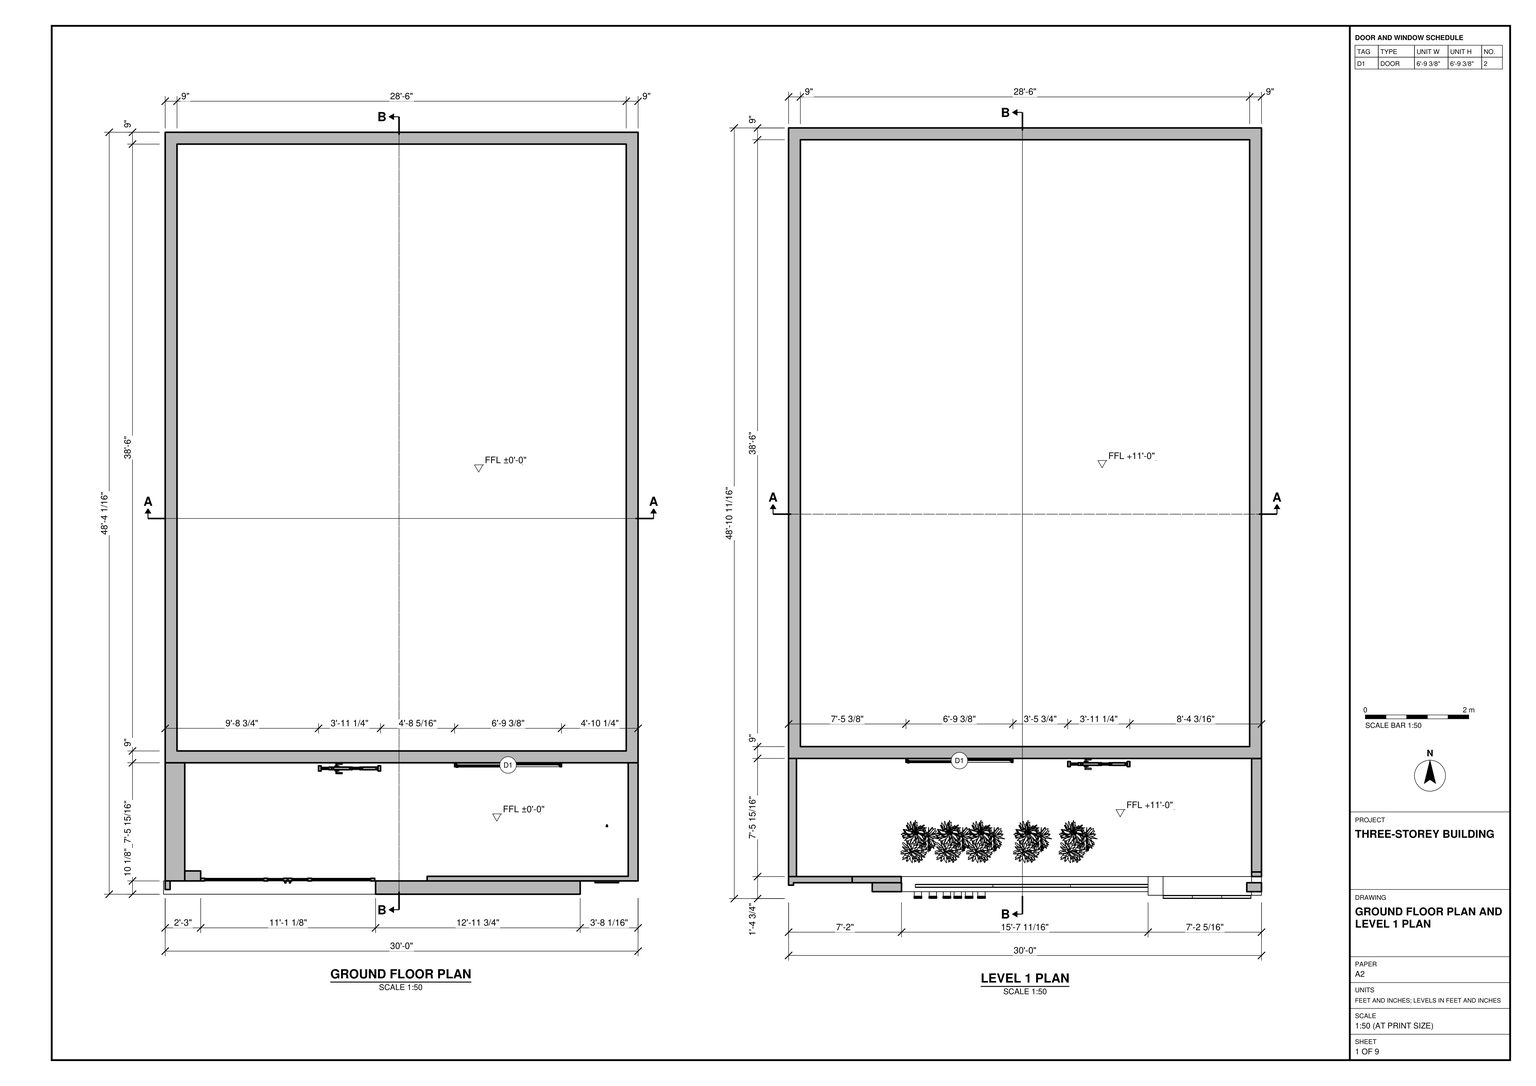
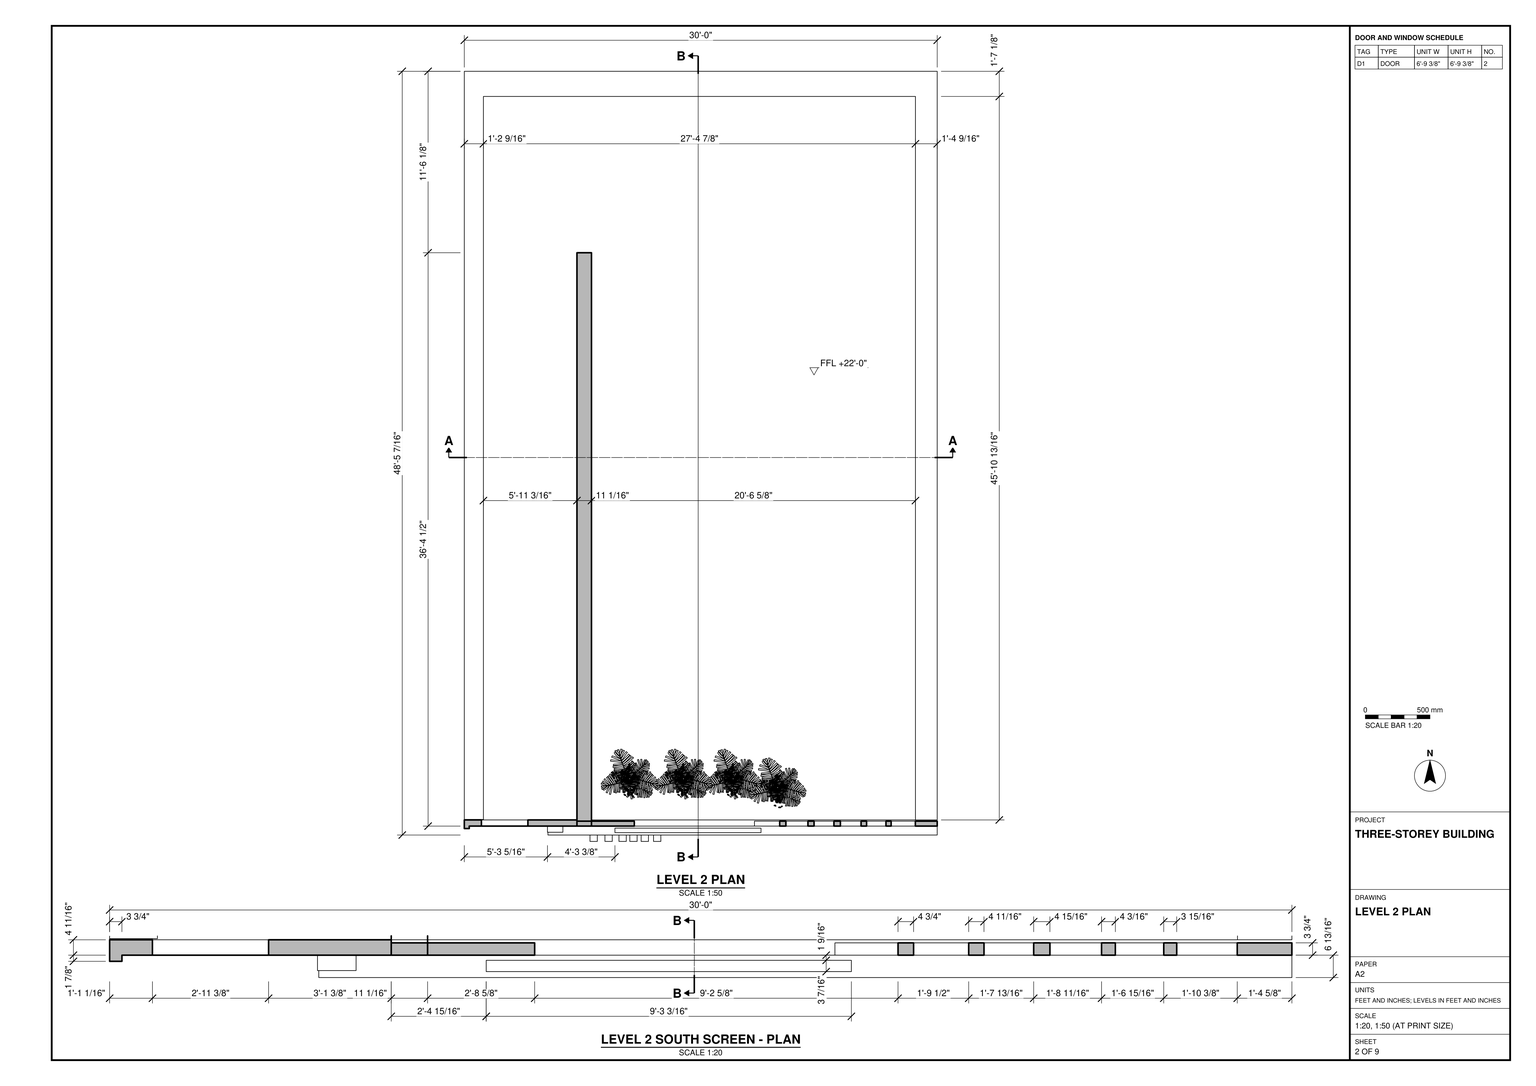
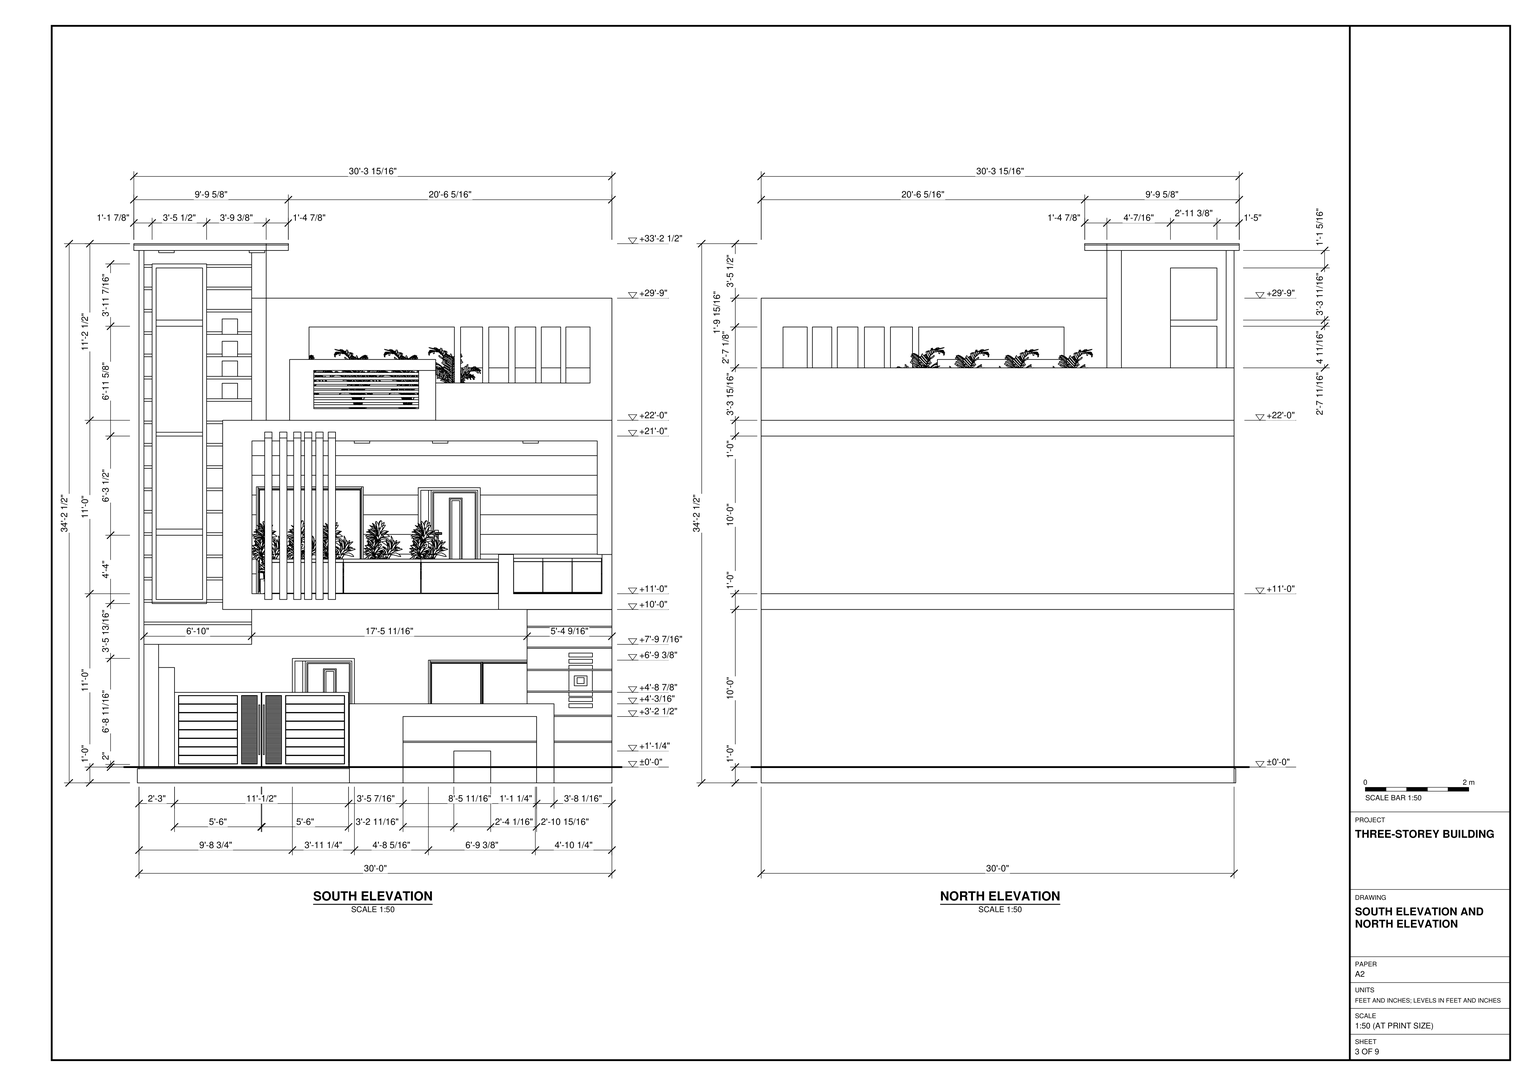
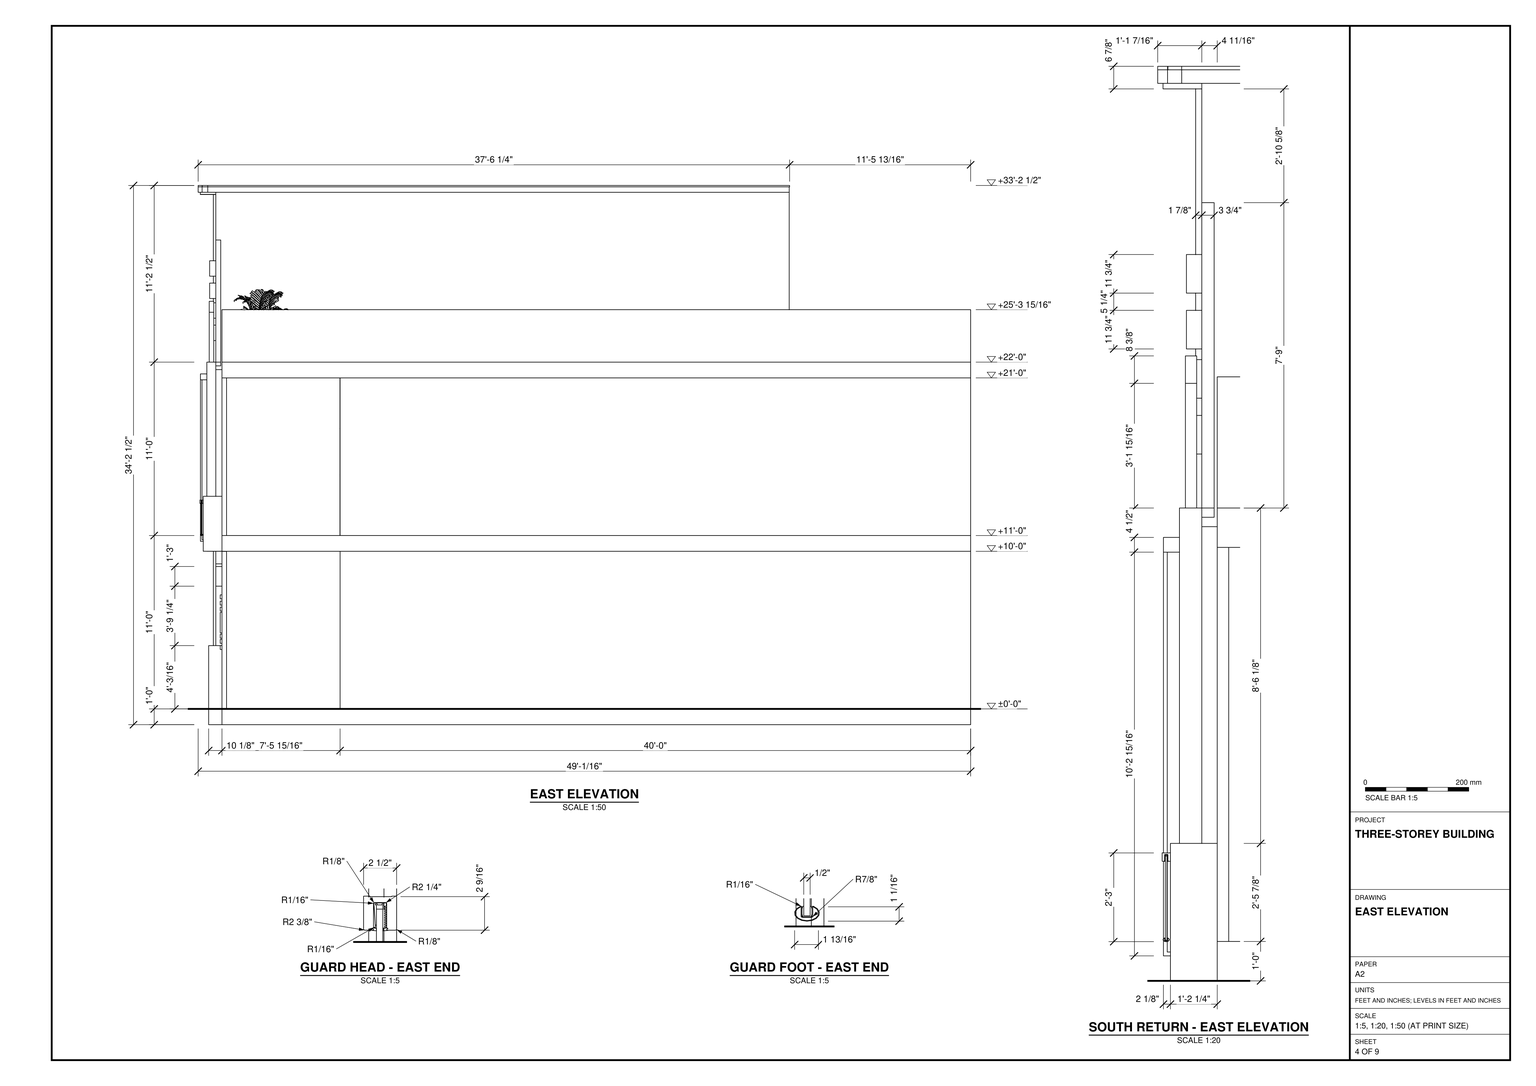
Build the three-storey building in SketchUp from task_files/diagram_01.pdf. Work in feet and inches. The overall model extents are 30'-3 15/16" wide, 49'-1/16" deep and 34'-2 1/2" high. Set the finished floor levels at ±0'-0", +11'-0" and +22'-0".

Use the plans to lay out the rectangular lower storeys with 9" perimeter walls and recessed outdoor spaces along the south side. Model the base, floor slabs and roof terrace with the edge profiles shown in elevation. At the ground-floor frontage, place the paired gate beside the low wall. Set the doors back from the gate line. The wide sliding door is on the right at ground level and on the left on the storey above when viewed from the south.

Build the projecting frame, railing and vertical fins around the first-floor balcony. On the roof terrace, include the offset longitudinal wall and the south screen with its wide opening, narrow slots and horizontal louvres. Match the tall capped bay at the west end of the south elevation. Decor and loose items, including the plants on the balcony and terrace, may be any suitable library components.

Keep shell elements such as walls, slabs and roof parts in separate groups or components, group each furniture or joinery piece separately, and use components for repeated parts. Save one SketchUp model as output_files/three_storey_building_with_a_screened_south_terrace.skp.

# SketchUp Ruby script. Lengths in inches.
U = 1.inch
M = Sketchup.active_model
def pt(a) = Geom::Point3d.new(a.map { |v| v * U })
def face(e, loops, mat)
  f = e.add_face(loops[0].map { |a| pt(a) })
  loops[1..].each { |l| e.add_face(l.map { |a| pt(a) }).erase! }
  f.material = f.back_material = mat if mat
  f
end
# faces: each face lists its corners as indices into pts; further lists are holes
def faces(e, pts, list, mat = nil) = list.each { |f| face(e, (f[0].is_a?(Array) ? f : [f]).map { |l| l.map { |i| pts[i] } }, mat) }
# xy, xz, yz: faces in a plane at the given z, y or x. An outline is a flat list of corners, or four numbers for a rectangle; further outlines are holes
def ring(l) = l.size == 4 ? [[l[0], l[1]], [l[2], l[1]], [l[2], l[3]], [l[0], l[3]]] : l.each_slice(2).to_a
def flat(e, list, mat, &to3) = list.each { |f| face(e, (f[0].is_a?(Array) ? f : [f]).map { |l| ring(l).map { |u, v| to3.(u, v) } }, mat) }
def xy(e, z, list, mat = nil) = flat(e, list, mat) { |x, y| [x, y, z] }
def xz(e, y, list, mat = nil) = flat(e, list, mat) { |x, z| [x, y, z] }
def yz(e, x, list, mat = nil) = flat(e, list, mat) { |y, z| [x, y, z] }
def lines(e, pts, list) = list.each { |a, b| e.add_line(pt(pts[a]), pt(pts[b])) }
# prism: a flat outline (further loops are holes) pulled along v
def prism(e, loops, v, mat = nil)
  f = face(e, loops, mat); d = Geom::Vector3d.new(v.map { |x| x * U })
  f.pushpull(f.normal.samedirection?(d) ? d.length : -d.length)
end
def box(e, o, s, mat = nil) = prism(e, [[o, [o[0] + s[0], o[1], o[2]], [o[0] + s[0], o[1] + s[1], o[2]], [o[0], o[1] + s[1], o[2]]]], [0, 0, s[2]], mat)
def at(x, y, z, deg = 0) = Geom::Transformation.translation(pt([x, y, z])) * Geom::Transformation.rotation(ORIGIN, Z_AXIS, deg.degrees)
def axes(o, x, y, z) = Geom::Transformation.new([*x, 0, *y, 0, *z, 0, *pt(o).to_a, 1])
def part(name) = M.definitions.add(name)
# library, detail: a bought-in or finely detailed component or shape, given as its bounding box
def library(name, o, s) = part(name).tap { |d| box(d.entities, o, s) }
def detail(e, o, s) = box(e.add_group.entities, o, s)
def put(e, d, t, mat = nil) = e.add_instance(d, t).tap { |i| i.material = mat if mat }
def group(e, t, mat = nil) = e.add_group.tap { |g| g.transformation = t; g.material = mat if mat }.entities
root = M.entities
M.materials.add("Glass_Tinted_Gray").color = [0, 0, 0]
M.materials["Glass_Tinted_Gray"].alpha = 0.125
M.materials.add("[0131_Silver]").color = [192, 192, 192]
M.materials.add("[0135_DarkGray]").color = [81, 81, 81]
M.materials.add("[Color C02]").color = [255, 204, 153]
M.materials.add("[Color C07]").color = [153, 76, 0]
M.materials.add("[Color D01]").color = [255, 242, 204]
M.materials.add("[Color E03]").color = [255, 255, 101]
M.materials.add("[Color F07]").color = [81, 104, 58]
M.materials.add("[Color M00]").color = [255, 255, 255]
M.materials.add("[Color M06]").color = [86, 86, 86]
M.materials.add("[Color M08]").color = [30, 30, 30]
M.materials.add("[Color M09]").color = [0, 0, 0]
M.materials.add("[Mirror 02]").color = [229, 229, 229]
M.materials.add("[Terrazzo Light Blue]").color = [196, 214, 227]
M.materials.add("[Translucent Glass Blue]").color = [100, 149, 237]
M.materials["[Translucent Glass Blue]"].alpha = 0.5
M.materials.add("[Wood Cherry Original]").color = [152, 86, 42]
c1 = library("ประตู",[99.61,0,0],[47.24,8.5625,80.71])
c2 = part("PENTEK_RP Fineline 50S_Sliding_DoorCase_E1")
box(c2.entities,[0,0,0],[1.51,3.66,99.27],"[0135_DarkGray]")
c3 = part("PENTEK_RP Fineline 50S_SlidingDooe_Case_E2")
box(c3.entities,[0,0,0],[96.25,3.66,1.51],"[0135_DarkGray]")
c4 = part("pentek_RP Fineline 50S_SlidingDoor_Case")
put(c4.entities,c2,at(97.76,0,0))
put(c4.entities,c3,at(1.51,0,0))
put(c4.entities,c2,at(0,0,0))
put(c4.entities,c3,at(1.51,0,97.76))
c5 = part("PENTEK_RP Fineline 50S_SlidingDoor_GlazingBead_2")
box(c5.entities,[0,0,0],[0.56,0.59,94.39],"[0135_DarkGray]")
c6 = part("PENTEK_RP Fineline 50S_SlidingDoor_Glass")
box(c6.entities,[0,0,0],[46.58,0.16,94.39],"Glass_Tinted_Gray")
c7 = part("PENTEK_RP Fineline 50S_SlidingDoor_GlazingBead")
box(c7.entities,[0,0,0],[45.47,0.59,0.56],"[0135_DarkGray]")
c8 = part("PENTEK_RP Fineline 50S_SlidingDoor_Leaf_E1")
xy(c8.entities,0,[[0,0,0.93,1.97],[0.93,1.57,1.49,1.97]],"[0135_DarkGray]")
xy(c8.entities,96.25,[[0,0,0.93,0,0.93,1.57,1.49,1.57,1.49,1.97,0,1.97]],"[0135_DarkGray]")
xz(c8.entities,0,[[0,0,0.93,96.25]],"[0135_DarkGray]")
xz(c8.entities,1.57,[[0.93,0,1.49,95.32],[0.93,95.32,1.49,96.25]],"[0135_DarkGray]")
xz(c8.entities,1.97,[[0,0,1.49,96.25]],"[0135_DarkGray]")
yz(c8.entities,0,[[0,0,1.97,96.25]],"[0135_DarkGray]")
yz(c8.entities,0.93,[[0,0,1.57,0.93],[0,0.93,1.57,95.32],[0,95.32,1.57,96.25]],"[0135_DarkGray]")
yz(c8.entities,1.49,[[1.57,0,1.97,95.32],[1.57,95.32,1.97,96.25]],"[0135_DarkGray]")
c9 = part("PENTEK_RP Fineline 50S_SlidingDoor_Leaf_E2")
xy(c9.entities,0,[[0,0,0,1.57,0.56,1.57,0.56,1.97,46.02,1.97,46.02,1.57,46.58,1.57,46.58,0]],"[0135_DarkGray]")
xy(c9.entities,0.93,[[0,0,46.58,1.57]],"[0135_DarkGray]")
xy(c9.entities,1.49,[[0.56,1.57,46.02,1.97]],"[0135_DarkGray]")
xz(c9.entities,0,[[0,0,46.58,0.93]],"[0135_DarkGray]")
xz(c9.entities,1.57,[[0,0,0.56,0.93],[46.02,0,46.58,0.93],[0.56,0.93,46.02,1.49]],"[0135_DarkGray]")
xz(c9.entities,1.97,[[0.56,0,46.02,1.49]],"[0135_DarkGray]")
yz(c9.entities,0,[[0,0,1.57,0.93]],"[0135_DarkGray]")
yz(c9.entities,0.56,[[1.57,0,1.97,0.93],[1.57,0.93,1.97,1.49]],"[0135_DarkGray]")
yz(c9.entities,46.02,[[1.57,0,1.97,0.93],[1.57,0.93,1.97,1.49]],"[0135_DarkGray]")
yz(c9.entities,46.58,[[0,0,1.57,0.93]],"[0135_DarkGray]")
c10 = part("PENTEK_RP Fineline S_SlidingDoor_Leaf1")
put(c10.entities,c5,at(0.93,0,0.93))
put(c10.entities,c5,at(46.96,0,0.93))
put(c10.entities,c6,at(1.49,1.42,0.93))
put(c10.entities,c7,at(1.49,0,0.93))
put(c10.entities,c6,at(1.49,0.59,0.93),"[Terrazzo Light Blue]")
put(c10.entities,c8,at(0,0,0))
put(c10.entities,c8,axes([48.44,0,0],[-1,0,0],[0,1,0],[0,0,1]))
put(c10.entities,c9,axes([0.93,0,96.25],[1,0,0],[0,1,0],[0,0,-1]))
put(c10.entities,c9,at(0.93,0,0))
put(c10.entities,c7,at(1.49,0,94.77))
c11 = part("PENTEK_RP Fineline 50S_SlidingDoor_Leaf2")
put(c11.entities,c6,at(1.49,1.42,0.93))
put(c11.entities,c7,at(1.49,0,94.77))
put(c11.entities,c5,at(46.96,0,0.93))
put(c11.entities,c6,at(1.49,0.59,0.93),"[Mirror 02]")
put(c11.entities,c5,at(0.93,0,0.93))
put(c11.entities,c8,at(0,0,0))
put(c11.entities,c8,axes([48.44,0,0],[-1,0,0],[0,1,0],[0,0,1]))
put(c11.entities,c7,at(1.49,0,0.93))
put(c11.entities,c9,axes([0.93,0,96.25],[1,0,0],[0,1,0],[0,0,-1]))
put(c11.entities,c9,at(0.93,0,0))
c12 = part("PENTEK - Slimmest Steel Sliding Door / Window\#1")
put(c12.entities,c4,at(0,-1.88,-0.09))
put(c12.entities,c10,at(1.51,-2.27,1.42))
put(c12.entities,c11,at(49.32,-0.3,1.42))
c13 = library("Wagner Glass Railing",[9.08,102.375,1.53],[2.51,145.5,42.05])
c14 = part("Gate+Design_02_ar+kalil")
p = [[0,0,0],[1,0,0],[1,1,0]]
lines(c14.entities,p,[[0,1],[1,2],[2,0]])
c15 = part("Gate leaf frame")
xy(c15.entities,0,[[[0,0,66,72],[3,3,48,69],[51,3,63,69]]])
xy(c15.entities,0.5,[[3,3,48,69]])
xy(c15.entities,1.5,[[3,3,48,11.25],[3,11.25,48,19.5],[3,19.5,48,27.75],[3,27.75,48,36],[3,36,48,44.25],
  [3,44.25,48,52.5],[3,52.5,48,60.75],[3,60.75,48,69]])
xy(c15.entities,2,[[[0,0,66,72],[3,3,48,69],[51,3,63,69]]])
xz(c15.entities,0,[[0,0,51,2],[51,0,66,2]])
xz(c15.entities,3,[[3,0,27,0.5],[27,0,48,0.5],[51,0,63,2],[3,1.5,48,2]])
xz(c15.entities,69,[[3,0,48,0.5],[51,0,63,2],[3,1.5,48,2]])
xz(c15.entities,72,[[0,0,66,2]])
yz(c15.entities,0,[[0,0,72,2]])
yz(c15.entities,3,[[3,0,69,0.5],[3,1.5,69,2]])
yz(c15.entities,48,[[3,0,69,0.5],[3,1.5,69,2]])
yz(c15.entities,51,[[3,0,69,2]])
yz(c15.entities,63,[[3,0,69,2]])
yz(c15.entities,66,[[0,0,72,2]])
c16 = part("Gate infill slat")
box(c16.entities,[0,0,0],[12,1,1])
c17 = part("Slatted gate infill")
put(c17.entities,c16,at(3,0.5,22.5))
put(c17.entities,c16,at(3,0.5,26.5))
put(c17.entities,c16,at(3,0.5,28.5))
put(c17.entities,c16,at(3,0.5,4.5))
put(c17.entities,c16,at(3,0.5,2.5))
put(c17.entities,c16,at(3,0.5,54.5))
put(c17.entities,c16,at(3,0.5,56.5))
put(c17.entities,c16,at(3,0.5,24.5))
put(c17.entities,c16,at(3,0.5,20.5))
put(c17.entities,c16,at(3,0.5,34.5))
put(c17.entities,c16,at(3,0.5,6.5))
put(c17.entities,c16,at(3,0.5,42.5))
put(c17.entities,c16,at(3,0.5,0.5))
put(c17.entities,c16,at(3,0.5,10.5))
put(c17.entities,c16,at(3,0.5,16.5))
put(c17.entities,c16,at(3,0.5,18.5))
put(c17.entities,c16,at(3,0.5,58.5))
put(c17.entities,c16,at(3,0.5,40.5))
put(c17.entities,c16,at(3,0.5,60.5))
put(c17.entities,c16,at(3,0.5,36.5))
put(c17.entities,c16,at(3,0.5,38.5))
put(c17.entities,c16,at(3,0.5,32.5))
put(c17.entities,c16,at(3,0.5,8.5))
put(c17.entities,c16,at(3,0.5,64.5))
put(c17.entities,c16,at(3,0.5,12.5))
put(c17.entities,c16,at(3,0.5,44.5))
put(c17.entities,c16,at(3,0.5,46.5))
put(c17.entities,c16,at(3,0.5,52.5))
put(c17.entities,c16,at(3,0.5,48.5))
put(c17.entities,c16,at(3,0.5,50.5))
put(c17.entities,c16,at(3,0.5,62.5))
put(c17.entities,c16,at(3,0.5,14.5))
put(c17.entities,c16,at(3,0.5,30.5))
c18 = part("Gate cladding strip")
xy(c18.entities,0.25,[[0.25,0,44.75,0.15]])
xy(c18.entities,8,[[0.25,0,44.75,0.15]])
xz(c18.entities,0,[[0.25,0.25,44.75,8]])
xz(c18.entities,0.15,[[[0,0,45,8.25],[0.25,0.25,44.75,8]]])
yz(c18.entities,0.25,[[0,0.25,0.15,8]])
yz(c18.entities,44.75,[[0,0.25,0.15,8]])
p = [[0,0.15,0],[0.25,0,0.25],[44.75,0,0.25],[45,0.15,0],[0,0.15,8.25],[0.25,0,8],
  [44.75,0,8],[45,0.15,8.25]]
faces(c18.entities,p,[[0,1,2,3],[4,5,1,0],[3,2,6,7],[5,4,7,6]])
c19 = part("Gate infill panel")
put(c19.entities,c18,at(0,0,24.75))
put(c19.entities,c18,at(0,0,57.75))
put(c19.entities,c18,at(0,0,49.5))
put(c19.entities,c18,at(0,0,41.25))
put(c19.entities,c18,at(0,0,33))
put(c19.entities,c18,axes([0,1.3,49.5],[1,0,0],[0,-1,0],[0,0,1]))
put(c19.entities,c18,at(0,0,16.5))
put(c19.entities,c18,at(0,0,8.25))
put(c19.entities,c18,axes([0,1.3,24.75],[1,0,0],[0,-1,0],[0,0,1]))
put(c19.entities,c18,at(0,0,0))
put(c19.entities,c18,axes([0,1.3,57.75],[1,0,0],[0,-1,0],[0,0,1]))
put(c19.entities,c18,axes([0,1.3,41.25],[1,0,0],[0,-1,0],[0,0,1]))
put(c19.entities,c18,axes([0,1.3,33],[1,0,0],[0,-1,0],[0,0,1]))
put(c19.entities,c18,axes([0,1.3,16.5],[1,0,0],[0,-1,0],[0,0,1]))
put(c19.entities,c18,axes([0,1.3,8.25],[1,0,0],[0,-1,0],[0,0,1]))
put(c19.entities,c18,axes([0,1.3,0],[1,0,0],[0,-1,0],[0,0,1]))
c20 = part("Gate leaf")
put(c20.entities,c15,axes([0,2,0],[1,0,0],[0,0,1],[0,-1,0]),"[0131_Silver]")
put(c20.entities,c17,at(48,0,3),"[0131_Silver]")
put(c20.entities,c19,at(3,0.35,3))
c21 = part("Gate pull handle")
prism(c21.entities,[[[0.35,0,3.8],[0.35,0,3],[0.35,-1.5,3],[0.35,-1.5,51],[0.35,0,51],[0.35,0,50.2],[0.35,-1,50.2],[0.35,-1,3.8]]],[0.8,0,0])
c22 = part("gate1")
put(c22.entities,c20,axes([145.27,6.5625,-22.58],[-1,0,0],[0,1,0],[0,0,1]))
put(c22.entities,c21,at(321.29,49.48,9),"[0131_Silver]")
put(c22.entities,c20,at(12.77,6.5625,-22.58))
put(c22.entities,c21,at(76.52,6.5625,-13.58),"[0131_Silver]")
put(c22.entities,c21,at(80.02,6.5625,-13.58),"[0131_Silver]")
c23 = library("KentiaPalm",[-22.86,-14.31,0],[47.49,43.96,59.125])
c24 = library("plant",[-35.72,-28.42,0],[66.31,67.39,84.38])
c25 = part("グループ\#88")
detail(c25.entities,[0,0,0],[11.8125,11.8125,1.69])
c26 = part("CL OL251733")
put(c26.entities,c25,axes([4.91,11.8125,72.56],[1,0,0],[0,-1,0],[0,0,-1]))
c27 = part("Group\#4")
box(c27.entities,[0,0,0],[5.5625,4.5,4.875])
c28 = part("Group\#5")
box(c28.entities,[0,0,0],[11.75,11.75,4.6875])
c29 = part("Group\#12")
box(c29.entities,[0,0,0],[2.125,2.125,85.0625])
prism(root,[[[3.9375,588.0625,264],[363.9375,588.0625,264],[363.9375,18.125,264],[347.375,18.125,264],[347.375,568.91,264],[18.48,568.91,264],[18.48,18.47,264],[3.9375,18.47,264]]],[0,0,39.9375])
xy(root,-12,[[2.67,8,204.92,18.125],[306.61,8,319.875,18.125],[243.61,15.8125,271.67,18.125]])
xy(root,0,[[3.9375,11.5625,7.6875,18.125],[3.9375,18.125,18.84,108.0625],[18.84,18.125,30.96,25.73],[203.36,18.125,363.9375,21.625],[356.42,21.625,363.9375,108.0625],
  [[3.9375,108.0625,363.9375,588.0625],[12.9375,117.0625,354.9375,579.0625]],[12.9375,117.0625,354.9375,579.0625]])
xy(root,12.25,[[243.61,15.8125,271.67,18.125]],"[Color C07]")
xy(root,38.52,[[204.92,8,306.61,18.125]])
xy(root,48.19,[[203.36,18.125,299.36,21.625]])
xy(root,48.19,[[164.11,8,319.875,18.125]],"[Color C07]")
xy(root,57.87,[[331.23,16.8125,349.06,18.125]])
xy(root,61.91,[[335.27,16.8125,345.01,18.125]])
xy(root,63.58,[[337.45,16.8125,342.76,18.125]])
xy(root,68.14,[[337.45,16.8125,342.76,18.125]])
xy(root,69.44,[[335.27,16.8125,345.01,18.125]])
xy(root,73.48,[[331.23,16.8125,349.06,18.125]])
xy(root,75.8125,[[18.84,18.125,30.96,25.73]],"[Color C07]")
xy(root,93.4375,[[7.6875,13.4375,7.6875,18.125,78.66,18.125,78.66,108.0625,89.69,108.0625,89.69,13.4375]])
xy(root,119.9,[[299.36,18.125,363.9375,21.625]])
xy(root,120,[[67.625,6.625,278.25,18.125],[3.9375,18.125,18.84,108.0625],[78.66,18.125,89.69,108.0625],[356.42,21.625,363.9375,108.0625],[[3.9375,108.0625,363.9375,588.0625],[12.9375,117.0625,354.9375,579.0625]]])
xy(root,120.02,[[277.62,3.875,363.9375,18.125]])
xy(root,127.58,[[16.97,13.4375,52.34,18.125]])
xy(root,127.61,[[99.61,1.75,105.18,6.625],[110.99,1.75,116.55,6.625],[121.68,1.75,127.24,6.625],[129.93,1.75,135.49,6.625],[138.55,1.75,144.11,6.625],
  [147.99,1.75,153.55,6.625]],"[Color M06]")
xy(root,128.78,[[99.61,2.91,105.18,6.625],[110.99,2.91,116.55,6.625],[121.68,2.91,127.24,6.625],[129.93,2.91,135.49,6.625],[138.55,2.91,144.11,6.625],
  [147.99,2.91,153.55,6.625]])
xy(root,131.9375,[[289.03,3.875,356.42,18.125]])
xy(root,132,[[89.92,6.625,278.25,6.625,278.25,18.125,67.625,18.125,67.625,13.4375,89.92,13.4375],[3.9375,18.125,9.95,108.0625],[356.42,18.125,363.9375,21.625],[356.42,21.625,363.9375,107.9375],[[3.9375,108.0625,363.9375,588.0625],[12.9375,117.0625,354.9375,579.0625]],
  [12.9375,117.0625,354.9375,579.0625]])
xy(root,161.86,[[277.62,3.875,289.03,18.125],[356.42,3.875,363.9375,6.625],[352.76,6.625,356.42,13.4375],[356.42,6.625,363.9375,13.4375],[356.42,13.4375,363.9375,18.125]])
xy(root,176.51,[[16.97,13.4375,52.34,18.125]])
xy(root,181.19,[[16.97,13.4375,52.34,18.125]])
xy(root,248.32,[[89.92,6.625,352.76,13.4375]],"[Wood Cherry Original]")
xy(root,250.55,[[99.61,1.75,105.18,2.91]])
xy(root,252,[[16.97,13.4375,52.34,18.125],[3.9375,18.125,9.95,108.0625],[356.42,18.125,363.9375,21.625],[356.42,21.625,363.9375,107.9375],[[3.9375,108.0625,363.9375,588.0625],[12.9375,117.0625,354.9375,579.0625]]])
xy(root,254.9,[[16.97,13.4375,52.34,18.125]])
xy(root,258.3125,[[89.69,13.4375,100.75,449.9375]])
xy(root,261.17,[[89.69,13.4375,133.36,17.1875]])
xy(root,264,[[[67.625,6.625,363.9375,13.4375],[118.61,8.4375,229.79,11.875]],[224.8,13.4375,363.9375,17.1875]])
xy(root,272.85,[[136.98,8.4375,216.82,11.875]],"[Color F07]")
xy(root,292.37,[[324.92,13.4375,328.87,17.1875],[328.87,13.4375,347.3,17.1875]])
xy(root,292.43,[[224.8,13.4375,244.01,17.1875],[244.01,13.4375,248.75,17.1875],[248.75,13.4375,265.52,17.1875],[265.52,13.4375,270.1875,17.1875],[270.1875,13.4375,285.3125,17.1875],
  [285.3125,13.4375,290.26,17.1875],[290.26,13.4375,305.98,17.1875],[305.98,13.4375,310.18,17.1875],[310.18,13.4375,324.92,17.1875]])
xy(root,301.96,[[216.82,8.4375,229.79,11.875]])
xy(root,301.96,[[136.98,8.4375,216.82,11.875]],"[Color F07]")
xy(root,310.3125,[[118.61,8.4375,229.79,11.875]],"[Color F07]")
xy(root,335.06,[[133.36,13.4375,244.01,17.1875],[248.75,13.4375,265.52,17.1875],[270.1875,13.4375,285.3125,17.1875],[290.26,13.4375,305.98,17.1875],[310.18,13.4375,324.92,17.1875],
  [328.87,13.4375,347.3,17.1875]])
xy(root,335.61,[[16.97,13.4375,52.34,18.125]])
xy(root,340.3,[[16.97,13.4375,52.34,18.125]])
xy(root,356.98,[[89.69,13.4375,363.9375,17.1875]])
xy(root,380,[[16.97,13.4375,52.34,18.125]])
xy(root,393.3125,[[0,11.5625,3.9375,13.4375],[3.9375,11.5625,7.6875,13.4375],[89.69,13.4375,100.75,449.9375]])
xy(root,393.3125,[[0,0,100.75,3],[100.75,0,117.63,3],[0,3,100.75,7.3125],[100.75,3,117.63,7.3125],[0,7.3125,0,11.5625,7.6875,11.5625,7.6875,13.4375,100.75,13.4375,100.75,7.3125],
  [100.75,7.3125,117.63,13.4375],[0,13.4375,3.9375,449.9375],[100.75,13.4375,117.63,449.9375],[3.9375,18.125,9.95,449.9375],[9.95,18.125,89.69,449.9375]],"[Color C07]")
xy(root,397.4375,[[0,0,100.75,3],[100.75,0,117.63,3],[0,3,100.75,7.3125],[100.75,3,103.75,3.125],[103.75,3,117.63,3.125],
  [100.75,3.125,117.63,7.3125],[0,7.3125,100.75,449.9375],[100.75,7.3125,117.63,449.9375],[117.63,7.3125,117.69,450.25],[100.75,449.9375,117.63,450.25]])
xy(root,398.5,[[100.75,3,103.75,3.125]])
xy(root,398.5,[[0,0,100.75,3],[100.75,0,117.63,3],[0,3,100.75,7.3125],[100.75,3.125,117.63,7.3125],[0,7.3125,100.75,449.9375],
  [100.75,7.3125,117.69,450.25]],"[Color C07]")
xz(root,0,[[0,393.3125,100.75,397.4375],[100.75,393.3125,117.63,397.4375],[0,397.4375,100.75,398.5],[100.75,397.4375,117.63,398.5]],"[Color C07]")
xz(root,1.75,[[99.61,127.61,105.18,250.55],[110.99,127.61,116.55,250.55],[121.68,127.61,127.24,250.55],[129.93,127.61,135.49,250.55],[138.55,127.61,144.11,250.55],
  [147.99,127.61,153.55,250.55]],"[Color M06]")
xz(root,2.91,[[99.61,128.78,105.18,250.55],[110.99,128.78,116.55,250.55],[121.68,128.78,127.24,250.55],[129.93,128.78,135.49,250.55],[138.55,128.78,144.11,250.55],
  [147.99,128.78,153.55,250.55]])
xz(root,3,[[0,393.3125,100.75,397.4375],[100.75,393.3125,117.63,397.4375],[0,397.4375,100.75,398.5],[100.75,397.4375,103.75,398.5],[103.75,397.4375,117.63,398.5]])
xz(root,3.125,[[103.75,397.4375,117.63,398.5]])
xz(root,3.875,[[277.62,120.02,363.9375,120.02,363.9375,161.86,356.42,161.86,356.42,131.9375,289.03,131.9375,289.03,161.86,277.62,161.86]])
xz(root,6.625,[[[67.625,120,278.25,120,278.25,132,89.92,132,89.92,248.32,352.76,248.32,352.76,161.86,363.9375,161.86,363.9375,264,67.625,264],[99.61,127.61,105.18,128.78],[121.68,127.61,127.24,128.78],[129.93,127.61,135.49,128.78],[138.55,127.61,144.11,128.78],[147.99,127.61,153.55,128.78]]],"[Color C07]")
xz(root,7.3125,[[0,393.3125,100.75,397.4375],[100.75,393.3125,117.63,397.4375],[0,397.4375,100.75,398.5],[100.75,397.4375,117.63,398.5],[117.63,397.4375,117.69,398.5]])
xz(root,8,[[164.11,-12,204.92,-12,204.92,38.52,306.61,38.52,306.61,-12,319.875,-12,319.875,48.19,164.11,48.19]],"[Color C07]")
xz(root,8.4375,[[[118.61,264,229.79,310.3125],[136.98,272.85,216.82,301.96]]],"[Color F07]")
xz(root,11.5625,[[3.9375,0,7.6875,393.3125]])
xz(root,11.875,[[[118.61,264,229.79,310.3125],[136.98,272.85,216.82,301.96]]],"[Color F07]")
xz(root,13.4375,[[7.6875,108.4375,89.69,110.4375],[7.6875,125.4375,13.91,127.4375],[55.41,125.4375,89.69,127.4375],[67.625,132,89.69,142.4375],[89.69,132,89.69,258.3125,100.75,258.3125,100.75,261.17,133.36,261.17,133.36,264,363.9375,264,363.9375,161.86,352.76,161.86,352.76,248.32,89.92,248.32,89.92,132],
  [7.6875,142.4375,13.91,144.4375],[55.41,142.4375,67.625,144.4375],[67.625,142.4375,89.69,144.4375],[67.625,144.4375,89.69,159.4375],[7.6875,159.4375,13.91,161.4375],
  [55.41,159.4375,67.625,161.4375],[67.625,159.4375,89.69,161.4375],[67.625,161.4375,89.69,176.4375],[7.6875,176.4375,13.91,178.4375],[55.41,176.4375,67.625,178.4375],
  [67.625,176.4375,89.69,178.4375],[67.625,178.4375,89.69,193.4375],[7.6875,193.4375,13.91,195.4375],[55.41,193.4375,67.625,195.4375],[67.625,193.4375,89.69,195.4375],
  [67.625,195.4375,89.69,210.4375],[7.6875,210.4375,13.91,212.4375],[55.41,210.4375,67.625,212.4375],[67.625,210.4375,89.69,212.4375],[67.625,212.4375,89.69,227.4375],
  [7.6875,227.4375,13.91,229.4375],[55.41,227.4375,67.625,229.4375],[67.625,227.4375,89.69,229.4375],[67.625,229.4375,89.69,244.4375],[7.6875,244.4375,13.91,246.4375],
  [55.41,244.4375,67.625,246.4375],[67.625,244.4375,89.69,246.4375],[67.625,246.4375,89.69,261.4375],[89.69,258.3125,100.75,261.17],[89.69,261.17,100.75,264],
  [100.75,261.17,133.36,264],[7.6875,261.4375,13.91,263.4375],[55.41,261.4375,67.625,263.4375],[67.625,261.4375,89.69,263.4375],[67.625,263.4375,89.69,264],
  [89.69,264,100.75,356.98],[[100.75,264,133.36,264,133.36,335.06,244.01,335.06,244.01,292.43,224.8,292.43,224.8,264,363.9375,264,363.9375,356.98,100.75,356.98],[290.26,292.43,290.26,335.06,305.98,335.06,305.98,292.43,310.18,292.43,310.18,335.06,324.92,335.06,324.92,292.43],[328.87,292.37,347.3,335.06],[248.75,292.43,265.52,335.06],[270.1875,292.43,285.3125,335.06]],[7.6875,278.4375,13.91,280.4375],[55.41,278.4375,89.69,280.4375],[7.6875,295.4375,13.91,297.4375],
  [55.41,295.4375,89.69,297.4375],[7.6875,312.4375,13.91,314.4375],[55.41,312.4375,89.69,314.4375],[7.6875,329.4375,13.91,331.4375],[55.41,329.4375,89.69,331.4375],
  [7.6875,346.4375,13.91,348.4375],[55.41,346.4375,89.69,348.4375],[7.6875,363.4375,13.91,365.4375],[55.41,363.4375,89.69,365.4375],[7.6875,380.4375,13.91,382.4375],
  [55.41,380.4375,89.69,382.4375]])
xz(root,13.4375,[[7.6875,93.4375,89.69,108.4375],[7.6875,110.4375,89.69,110.4375,89.69,125.4375,55.41,125.4375,55.41,124.51,13.91,124.51,13.91,125.4375,7.6875,125.4375],[7.6875,127.4375,13.91,142.4375],[55.41,127.4375,89.69,127.4375,89.69,132,67.625,132,67.625,142.4375,55.41,142.4375],[7.6875,144.4375,13.91,159.4375],
  [55.41,144.4375,67.625,159.4375],[7.6875,161.4375,13.91,176.4375],[55.41,161.4375,67.625,176.4375],[7.6875,178.4375,13.91,193.4375],[55.41,178.4375,67.625,193.4375],
  [7.6875,195.4375,13.91,210.4375],[55.41,195.4375,67.625,210.4375],[7.6875,212.4375,13.91,227.4375],[55.41,212.4375,67.625,227.4375],[7.6875,229.4375,13.91,244.4375],
  [55.41,229.4375,67.625,244.4375],[7.6875,246.4375,13.91,261.4375],[55.41,246.4375,67.625,261.4375],[7.6875,263.4375,13.91,278.4375],[55.41,263.4375,67.625,263.4375,67.625,264,89.69,264,89.69,278.4375,55.41,278.4375],
  [7.6875,280.4375,13.91,295.4375],[55.41,280.4375,89.69,295.4375],[7.6875,297.4375,13.91,312.4375],[55.41,297.4375,89.69,312.4375],[7.6875,314.4375,13.91,329.4375],
  [55.41,314.4375,89.69,329.4375],[7.6875,331.4375,13.91,346.4375],[55.41,331.4375,89.69,346.4375],[7.6875,348.4375,13.91,363.4375],[55.41,348.4375,89.69,363.4375],
  [89.69,356.98,100.75,393.3125],[7.6875,365.4375,13.91,380.4375],[55.41,365.4375,89.69,380.4375],[7.6875,382.4375,13.91,382.4375,13.91,383.07,55.41,383.07,55.41,382.4375,89.69,382.4375,89.69,393.3125,7.6875,393.3125]],"[Color F07]")
xz(root,13.4375,[[[13.91,125.4375,55.41,383.07],[16.97,127.58,52.34,380]]],"[Color M00]")
xz(root,13.4375,[[13.91,124.51,55.41,125.4375],[16.97,176.51,52.34,181.19],[16.97,252,52.34,254.9],[16.97,335.61,52.34,340.3]],"[Color M09]")
xz(root,13.4375,[[16.97,127.58,52.34,176.51],[16.97,181.19,52.34,252],[16.97,254.9,52.34,335.61],[16.97,340.3,52.34,380]],"[Translucent Glass Blue]")
xz(root,15.8125,[[243.61,-12,271.67,12.25]],"[Color C07]")
xz(root,16.8125,[[[331.23,57.87,349.06,73.48],[335.27,61.91,345.01,69.44]]],"[Color D01]")
xz(root,16.8125,[[337.45,63.58,342.76,68.14]],"[Color E03]")
xz(root,17.1875,[[[89.69,261.17,89.69,356.98,363.9375,356.98,363.9375,264,224.8,264,224.8,292.43,244.01,292.43,244.01,335.06,133.36,335.06,133.36,261.17],[290.26,292.43,324.92,292.43,324.92,335.06,310.18,335.06,310.18,292.43,305.98,292.43,305.98,335.06,290.26,335.06],[328.87,292.37,347.3,335.06],[248.75,292.43,265.52,335.06],[270.1875,292.43,285.3125,335.06]]])
xz(root,18.125,[[2.67,-12,2.67,-1.16,164.11,-1.16,164.11,39.52,203.36,39.52,203.36,0,204.92,0,204.92,-12],[243.61,-12,271.67,0],[306.61,-12,319.875,0],[3.9375,0,3.9375,120,9.95,120,9.95,93.4375,7.6875,93.4375,7.6875,0],[203.36,0,204.92,18.76],
  [243.61,0,271.67,12.25],[306.61,0,319.875,18.76],[203.36,18.76,204.92,19.76],[204.92,18.76,306.61,19.76],[306.61,18.76,319.875,19.76],
  [319.875,18.76,363.9375,19.76],[203.36,19.76,204.92,38.52],[306.61,19.76,319.875,38.52],[203.36,38.52,319.875,39.52],[319.875,38.52,363.9375,39.52],
  [164.11,39.52,203.36,48.19],[203.36,39.52,319.875,48.19],[299.36,56.87,363.9375,57.87],[[335.27,61.91,345.01,69.44],[337.45,63.58,342.76,68.14]],[299.36,73.48,363.9375,74.48],
  [299.36,90.375,363.9375,91.375],[9.95,93.4375,18.84,120],[[18.84,93.4375,18.84,120,9.95,120,9.95,393.3125,89.69,393.3125,89.69,132,67.625,132,67.625,120,78.66,120,78.66,93.4375],[16.97,254.9,52.34,335.61],[16.97,181.19,52.34,252],[16.97,127.58,52.34,176.51],[16.97,340.3,52.34,380]],[299.36,106.25,363.9375,107.25],[306.61,119.9,349.81,120],
  [349.81,119.9,363.9375,120.02],[3.9375,120,9.95,132],[67.625,120,89.69,132],[89.69,120,89.69,132,277.62,132,277.62,120.02,278.25,120.02,278.25,120],[306.61,120,349.81,120.02],
  [277.62,120.02,278.25,132],[278.25,120.02,278.25,132,277.62,132,277.62,161.86,289.03,161.86,289.03,131.9375,356.42,131.9375,356.42,132,363.9375,132,363.9375,120.02],[3.9375,132,9.95,252],[356.42,132,363.9375,161.86],[356.42,161.86,363.9375,252],
  [3.9375,252,9.95,393.3125]])
xz(root,18.125,[[18.84,0,30.96,75.8125]],"[Color C07]")
xz(root,18.125,[[7.6875,0,18.84,93.4375],[204.92,0,243.61,0,243.61,12.25,271.67,12.25,271.67,0,306.61,0,306.61,18.76,204.92,18.76],[319.875,0,363.9375,18.76],[204.92,19.76,306.61,38.52],[319.875,19.76,363.9375,38.52],
  [319.875,39.52,363.9375,39.52,363.9375,56.87,299.36,56.87,299.36,48.19,319.875,48.19],[299.36,57.87,331.23,73.48],[349.06,57.87,363.9375,73.48],[299.36,74.48,363.9375,90.375],[299.36,91.375,363.9375,106.25],
  [299.36,107.25,363.9375,119.9]],"[Color F07]")
xz(root,21.625,[[203.36,0,203.36,48.19,299.36,48.19,299.36,119.9,356.42,119.9,356.42,0],[356.42,119.9,363.9375,120],[356.42,132,363.9375,252]])
xz(root,25.73,[[18.84,0,30.96,75.8125]])
xz(root,107.9375,[[356.42,132,363.9375,252]])
xz(root,108.0625,[[3.9375,0,18.84,120],[18.84,0,356.42,0,356.42,120,89.69,120,89.69,93.4375,78.66,93.4375,78.66,120,18.84,120],[356.42,0,363.9375,120],[3.9375,132,9.95,252],[9.95,132,363.9375,252]])
xz(root,117.0625,[[12.9375,0,354.9375,120],[12.9375,132,354.9375,252]])
xz(root,449.9375,[[89.69,258.3125,100.75,393.3125]])
xz(root,449.9375,[[0,393.3125,100.75,397.4375],[100.75,393.3125,117.63,397.4375],[0,397.4375,100.75,398.5]],"[Color C07]")
xz(root,450.25,[[100.75,397.4375,117.69,398.5]],"[Color C07]")
xz(root,579.0625,[[12.9375,0,354.9375,120],[12.9375,132,354.9375,252]])
xz(root,588.0625,[[3.9375,0,363.9375,120],[3.9375,132,363.9375,252]])
yz(root,0,[[0,393.3125,3,397.4375],[3,393.3125,7.3125,397.4375],[7.3125,393.3125,449.9375,397.4375],[0,397.4375,3,398.5],[3,397.4375,7.3125,398.5],
  [7.3125,397.4375,449.9375,398.5]],"[Color C07]")
yz(root,2.67,[[8,-12,18.125,-1.16,18.125,-12]])
yz(root,3.9375,[[11.5625,0,18.125,393.3125],[18.125,0,108.0625,120],[108.0625,0,588.0625,120],[18.125,132,108.0625,252],[108.0625,132,588.0625,252]])
yz(root,7.6875,[[11.5625,0,13.4375,1.67],[13.4375,0,18.125,1.67],[11.5625,1.67,13.4375,393.3125],[13.4375,1.67,18.125,93.4375]])
yz(root,9.95,[[18.125,132,108.0625,252]])
yz(root,12.9375,[[117.0625,0,579.0625,120],[117.0625,132,579.0625,252]])
yz(root,16.97,[[13.4375,127.58,18.125,176.51],[13.4375,181.19,18.125,252],[13.4375,254.9,18.125,335.61],[13.4375,340.3,18.125,380]])
yz(root,18.84,[[18.125,0,25.73,75.8125]])
yz(root,18.84,[[25.73,0,108.0625,0,108.0625,120,18.125,120,18.125,75.8125,25.73,75.8125]],"[Color C02]")
yz(root,30.96,[[18.125,0,25.73,75.8125]],"[Color C07]")
yz(root,52.34,[[13.4375,127.58,18.125,176.51],[13.4375,176.51,18.125,181.19],[13.4375,181.19,18.125,252],[13.4375,252,18.125,254.9],[13.4375,254.9,18.125,304.41],
  [13.4375,304.41,18.125,335.61],[13.4375,335.61,18.125,340.3],[13.4375,340.3,18.125,380]])
yz(root,67.625,[[6.625,120,6.625,264,13.4375,264,13.4375,132,18.125,132,18.125,120]])
yz(root,78.66,[[18.125,93.4375,108.0625,120]])
yz(root,89.69,[[13.4375,108.4375,108.0625,110.4375],[18.125,258.3125,449.9375,393.3125],[13.4375,261.17,17.1875,356.98],[17.1875,261.17,18.125,278.23]])
yz(root,89.69,[[13.4375,93.4375,108.0625,108.4375],[13.4375,110.4375,108.0625,110.4375,108.0625,120,18.125,120,18.125,258.3125,13.4375,258.3125],[13.4375,258.3125,18.125,261.17],[17.1875,278.23,17.1875,356.98,13.4375,356.98,13.4375,393.3125,18.125,393.3125,18.125,278.23]],"[Color F07]")
yz(root,89.92,[[6.625,132,13.4375,248.32]])
yz(root,99.61,[[1.75,127.61,1.75,250.55,2.91,250.55,2.91,128.78,6.625,128.78,6.625,127.61]])
yz(root,100.75,[[0,393.3125,3,397.4375],[3,393.3125,7.3125,397.4375],[7.3125,393.3125,449.9375,397.4375],[0,397.4375,3,398.5],[3,397.4375,3.125,398.5],
  [3.125,397.4375,7.3125,398.5],[7.3125,397.4375,449.9375,398.5],[449.9375,397.4375,450.25,398.5]])
yz(root,100.75,[[13.4375,258.3125,449.9375,393.3125]],"[Color F07]")
yz(root,103.75,[[3,397.4375,3.125,398.5]])
yz(root,105.18,[[1.75,127.61,6.625,127.61,6.625,128.78,2.91,128.78,2.91,250.55,1.75,250.55]],"[Color M06]")
yz(root,110.99,[[1.75,127.61,1.75,250.55,2.91,250.55,2.91,128.78,6.625,128.78,6.625,127.61]])
yz(root,116.55,[[1.75,127.61,6.625,127.61,6.625,128.78,2.91,128.78,2.91,250.55,1.75,250.55]],"[Color M06]")
yz(root,117.63,[[0,393.3125,3,397.4375],[3,393.3125,7.3125,397.4375],[7.3125,393.3125,449.9375,397.4375],[0,397.4375,3,398.5],[3.125,397.4375,7.3125,398.5]],"[Color C07]")
yz(root,117.69,[[7.3125,397.4375,450.25,398.5]],"[Color C07]")
yz(root,118.61,[[8.4375,264,11.875,310.3125]],"[Color F07]")
yz(root,121.68,[[1.75,127.61,1.75,250.55,2.91,250.55,2.91,128.78,6.625,128.78,6.625,127.61]])
yz(root,127.24,[[1.75,127.61,6.625,127.61,6.625,128.78,2.91,128.78,2.91,250.55,1.75,250.55]],"[Color M06]")
yz(root,129.93,[[1.75,127.61,1.75,250.55,2.91,250.55,2.91,128.78,6.625,128.78,6.625,127.61]])
yz(root,133.36,[[13.4375,261.17,17.1875,335.06]])
yz(root,135.49,[[1.75,127.61,6.625,127.61,6.625,128.78,2.91,128.78,2.91,250.55,1.75,250.55]],"[Color M06]")
yz(root,136.98,[[8.4375,272.85,11.875,301.96]],"[Color F07]")
yz(root,138.55,[[1.75,127.61,1.75,250.55,2.91,250.55,2.91,128.78,6.625,128.78,6.625,127.61]])
yz(root,144.11,[[1.75,127.61,6.625,127.61,6.625,128.78,2.91,128.78,2.91,250.55,1.75,250.55]],"[Color M06]")
yz(root,147.99,[[1.75,127.61,1.75,250.55,2.91,250.55,2.91,128.78,6.625,128.78,6.625,127.61]])
yz(root,153.55,[[1.75,127.61,6.625,127.61,6.625,128.78,2.91,128.78,2.91,250.55,1.75,250.55]],"[Color M06]")
yz(root,164.11,[[8,-12,8,48.19,18.125,48.19,18.125,-1.16]])
yz(root,203.36,[[18.125,0,21.625,48.19]])
yz(root,204.92,[[8,-12,18.125,38.52]],"[Color C07]")
yz(root,216.82,[[8.4375,272.85,11.875,301.96]],"[Color F07]")
yz(root,224.8,[[13.4375,264,17.1875,292.43]])
yz(root,229.79,[[8.4375,264,11.875,301.96],[8.4375,301.96,11.875,310.3125]],"[Color F07]")
yz(root,243.61,[[15.8125,-12,18.125,12.25]],"[Color C07]")
yz(root,244.01,[[13.4375,292.43,17.1875,335.06]])
yz(root,248.75,[[13.4375,292.43,17.1875,335.06]])
yz(root,265.52,[[13.4375,292.43,17.1875,335.06]])
yz(root,270.1875,[[13.4375,292.43,17.1875,335.06]])
yz(root,271.67,[[15.8125,-12,18.125,12.25]],"[Color C07]")
yz(root,277.62,[[3.875,120.02,18.125,161.86]])
yz(root,278.25,[[6.625,120,18.125,132]])
yz(root,285.3125,[[13.4375,292.43,17.1875,335.06]])
yz(root,289.03,[[3.875,131.9375,18.125,161.86]])
yz(root,290.26,[[13.4375,292.43,17.1875,335.06]])
yz(root,299.36,[[18.125,48.19,21.625,119.9]])
yz(root,305.98,[[13.4375,292.43,17.1875,335.06]])
yz(root,306.61,[[8,-12,18.125,38.52]],"[Color C07]")
yz(root,310.18,[[13.4375,292.43,17.1875,335.06]])
yz(root,319.875,[[8,-12,18.125,48.19]],"[Color C07]")
yz(root,324.92,[[13.4375,292.37,17.1875,292.43],[13.4375,292.43,17.1875,335.06]])
yz(root,328.87,[[13.4375,292.37,17.1875,335.06]])
yz(root,331.23,[[16.8125,57.87,18.125,73.48]])
yz(root,335.27,[[16.8125,61.91,18.125,69.44]])
yz(root,337.45,[[16.8125,63.58,18.125,68.14]])
yz(root,342.76,[[16.8125,63.58,18.125,68.14]])
yz(root,345.01,[[16.8125,61.91,18.125,69.44]])
yz(root,347.3,[[13.4375,292.37,17.1875,335.06]])
yz(root,349.06,[[16.8125,57.87,18.125,73.48]])
yz(root,352.76,[[6.625,161.86,13.4375,248.32]])
yz(root,354.9375,[[117.0625,0,579.0625,120],[117.0625,132,579.0625,252]])
yz(root,356.42,[[21.625,0,108.0625,120],[3.875,131.9375,18.125,161.86],[18.125,132,21.625,252],[21.625,132,107.9375,252]])
yz(root,363.9375,[[18.125,0,21.625,119.9],[21.625,0,108.0625,120],[108.0625,0,588.0625,120],[3.875,120.02,18.125,161.86],[18.125,132,21.625,252],
  [21.625,132,107.9375,252],[108.0625,132,588.0625,252],[6.625,161.86,13.4375,264],[13.4375,264,17.1875,356.98]])
p = [[164.11,8,-12],[164.11,18.125,-1.16],[2.67,18.125,-1.16],[2.67,8,-12],[13.91,16.5,331.4375],[7.6875,16.5,331.4375],
  [9.95,108.0625,237.125],[356.42,108.0625,237.125],[9.95,108.0625,222.125],[356.42,108.0625,222.125],[9.95,108.0625,207.125],[356.42,108.0625,207.125],
  [9.95,108.0625,192.125],[356.42,108.0625,192.125],[9.95,108.0625,177.125],[356.42,108.0625,177.125],[9.95,108.0625,162.125],[356.42,108.0625,162.125],
  [9.95,108.0625,147.125],[356.42,108.0625,147.125],[306.61,21.625,48.19],[306.61,21.8125,48.19]]
faces(root,p,[[0,1,2,3]])
lines(root,p,[[4,5],[6,7],[8,9],[10,11],[12,13],[14,15],[16,17],[18,19],[20,21]])
put(root,c1,at(116.87,99.5,132))
put(root,c1,at(21.07,99.5,2.01))
put(root,c12,axes([93.29,106.6,132.07],[0.82,0,0],[0,0.82,0],[0,0,0.82]))
put(root,c13,axes([241.94,12.95,159.99],[0,-1,0],[0.46,0,0],[0,0,-0.64366]))
put(root,c13,axes([-24.27,21.38,159.35],[0,-1,0],[1.21791,0,0],[0,0,-0.64366]))
put(root,c14,at(-280.79,18.125,0))
put(root,c22,axes([18.19,11.5625,17.83],[1,0,0],[0,1,0],[0,0,0.79]))
put(root,c12,axes([224.25,106.6,0.07],[0.82,0,0],[0,0.82,0],[0,0,0.82]))
put(root,c23,at(129.14,45.28,262.64))
put(root,c23,at(170.08,45.28,262.64))
put(root,c23,at(207.89,45.28,262.64))
put(root,c23,at(241.75,38.6,264))
put(root,c24,axes([102.48,41.46,132],[0.66,0,0],[0,0.66,0],[0,0,0.66]))
put(root,c24,axes([128.48,41.46,132],[0.66,0,0],[0,0.66,0],[0,0,0.66]))
put(root,c24,axes([152.42,41.46,132],[0.66,0,0],[0,0.66,0],[0,0,0.66]))
put(root,c24,axes([188.23,41.46,132],[0.66,0,0],[0,0.66,0],[0,0,0.66]))
put(root,c24,axes([222.85,41.46,132],[0.66,0,0],[0,0.66,0],[0,0,0.66]))
put(root,c26,at(291.26,39.55,175.76))
put(root,c26,at(222.38,39.55,175.76))
put(root,c26,at(162.88,39.55,175.76))
put(root,c26,at(14.03,1.625,320.75))
put(root,c26,at(82.91,1.625,320.75))
g1 = group(root,at(3.9375,588.0625,-12),"[Color F07]")
box(g1,[0,-569.9375,0],[360,569.9375,12])
g2 = group(root,at(3.9375,588.0625,120))
box(g2,[0,-569.9375,0],[360,569.9375,12])
g3 = group(root,at(3.9375,588.0625,252),"[Color M00]")
box(g3,[0,-569.9375,0],[360,569.9375,12])
put(root,c27,axes([99.61,6.625,250.55],[1,0,0],[0,0,1],[0,-1,0]),"[Color M06]")
put(root,c27,axes([110.99,6.625,250.55],[1,0,0],[0,0,1],[0,-1,0]),"[Color M06]")
put(root,c27,axes([121.68,6.625,250.55],[1,0,0],[0,0,1],[0,-1,0]),"[Color M06]")
put(root,c27,axes([129.93,6.625,250.55],[1,0,0],[0,0,1],[0,-1,0]),"[Color M06]")
put(root,c27,axes([138.55,6.625,250.55],[1,0,0],[0,0,1],[0,-1,0]),"[Color M06]")
put(root,c27,axes([147.99,6.625,250.55],[1,0,0],[0,0,1],[0,-1,0]),"[Color M06]")
put(root,c28,axes([67.23,13.4375,280.4375],[1,0,0],[0,0,1],[0,-1,0]))
put(root,c28,axes([67.23,13.4375,297.4375],[1,0,0],[0,0,1],[0,-1,0]))
put(root,c28,axes([67.23,13.4375,312.4375],[1,0,0],[0,0,1],[0,-1,0]))
put(root,c28,axes([67.23,13.4375,329.4375],[1,0,0],[0,0,1],[0,-1,0]))
g4 = group(root,at(331.21,18.125,74.48),"[Color D01]")
box(g4,[0,-1.3125,0],[17.9375,1.3125,3])
g5 = group(root,at(331.21,18.125,79.05),"[Color D01]")
box(g5,[0,-1.3125,0],[17.9375,1.3125,3])
g6 = group(root,at(331.21,18.125,83.8125),"[Color D01]")
box(g6,[0,-1.3125,0],[17.9375,1.3125,3])
g7 = group(root,at(331.21,18.125,53.87),"[Color D01]")
box(g7,[0,-1.3125,0],[17.9375,1.3125,3])
g8 = group(root,at(331.21,18.125,49.93),"[Color D01]")
box(g8,[0,-1.3125,0],[17.9375,1.3125,3])
g9 = group(root,at(331.21,18.125,45.25),"[Color D01]")
box(g9,[0,-1.3125,0],[17.9375,1.3125,3])
put(root,c29,axes([136.98,9.05,273.76],[0,1,0],[0,0,1],[1,0,0]),"[Color M08]")
put(root,c29,axes([136.98,9.05,277.57],[0,1,0],[0,0,1],[1,0,0]),"[Color M08]")
put(root,c29,axes([136.98,9.05,281.44],[0,1,0],[0,0,1],[1,0,0]),"[Color M08]")
put(root,c29,axes([136.98,9.05,284.76],[0,1,0],[0,0,1],[1,0,0]),"[Color M08]")
put(root,c29,axes([136.98,9.05,288.01],[0,1,0],[0,0,1],[1,0,0]),"[Color M08]")
put(root,c29,axes([136.98,9.05,291.38],[0,1,0],[0,0,1],[1,0,0]),"[Color M08]")
put(root,c29,axes([136.98,9.05,294.82],[0,1,0],[0,0,1],[1,0,0]),"[Color M08]")
put(root,c29,axes([136.98,9.05,298.26],[0,1,0],[0,0,1],[1,0,0]),"[Color M08]")
